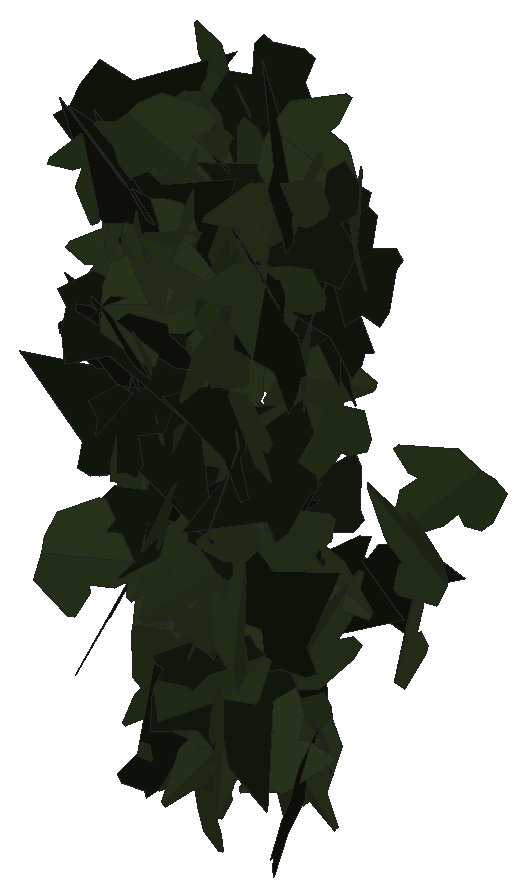
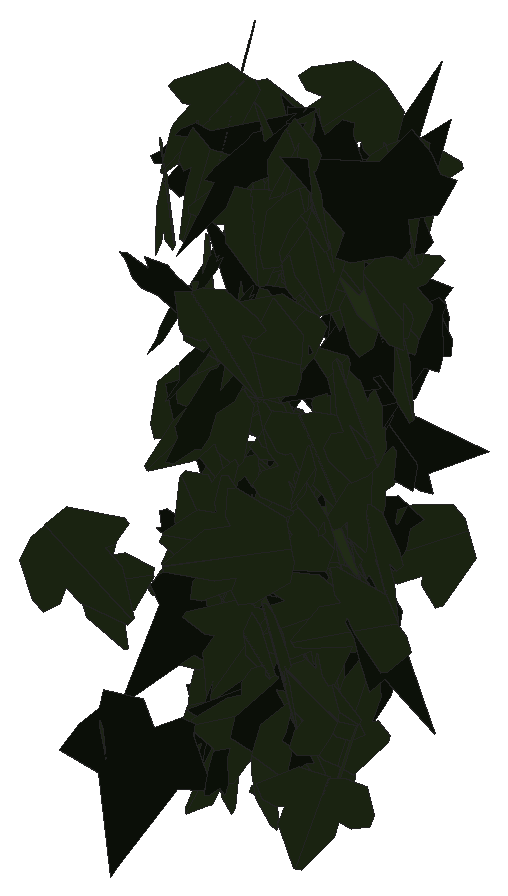
# SketchUp Ruby script. Lengths in inches.
U = 1.inch
M = Sketchup.active_model
def pt(a) = Geom::Point3d.new(a.map { |v| v * U })
def face(e, loops, mat)
  f = e.add_face(loops[0].map { |a| pt(a) })
  loops[1..].each { |l| e.add_face(l.map { |a| pt(a) }).erase! }
  f.material = f.back_material = mat if mat
  f
end
# faces: each face lists its corners as indices into pts; further lists are holes
def faces(e, pts, list, mat = nil) = list.each { |f| face(e, (f[0].is_a?(Array) ? f : [f]).map { |l| l.map { |i| pts[i] } }, mat) }
# xy, xz, yz: faces in a plane at the given z, y or x. An outline is a flat list of corners, or four numbers for a rectangle; further outlines are holes
def ring(l) = l.size == 4 ? [[l[0], l[1]], [l[2], l[1]], [l[2], l[3]], [l[0], l[3]]] : l.each_slice(2).to_a
def flat(e, list, mat, &to3) = list.each { |f| face(e, (f[0].is_a?(Array) ? f : [f]).map { |l| ring(l).map { |u, v| to3.(u, v) } }, mat) }
def xy(e, z, list, mat = nil) = flat(e, list, mat) { |x, y| [x, y, z] }
def xz(e, y, list, mat = nil) = flat(e, list, mat) { |x, z| [x, y, z] }
def yz(e, x, list, mat = nil) = flat(e, list, mat) { |y, z| [x, y, z] }
def lines(e, pts, list) = list.each { |a, b| e.add_line(pt(pts[a]), pt(pts[b])) }
# prism: a flat outline (further loops are holes) pulled along v
def prism(e, loops, v, mat = nil)
  f = face(e, loops, mat); d = Geom::Vector3d.new(v.map { |x| x * U })
  f.pushpull(f.normal.samedirection?(d) ? d.length : -d.length)
end
def box(e, o, s, mat = nil) = prism(e, [[o, [o[0] + s[0], o[1], o[2]], [o[0] + s[0], o[1] + s[1], o[2]], [o[0], o[1] + s[1], o[2]]]], [0, 0, s[2]], mat)
def at(x, y, z, deg = 0) = Geom::Transformation.translation(pt([x, y, z])) * Geom::Transformation.rotation(ORIGIN, Z_AXIS, deg.degrees)
def axes(o, x, y, z) = Geom::Transformation.new([*x, 0, *y, 0, *z, 0, *pt(o).to_a, 1])
def part(name) = M.definitions.add(name)
# library, detail: a bought-in or finely detailed component or shape, given as its bounding box
def library(name, o, s) = part(name).tap { |d| box(d.entities, o, s) }
def detail(e, o, s) = box(e.add_group.entities, o, s)
def put(e, d, t, mat = nil) = e.add_instance(d, t).tap { |i| i.material = mat if mat }
def group(e, t, mat = nil) = e.add_group.tap { |g| g.transformation = t; g.material = mat if mat }.entities
root = M.entities
M.materials.add("efeu1").color = [18, 25, 13]
M.materials.add("efeu2").color = [43, 57, 29]
c1 = part("ivyleaf_9")
p = [[1.54,2.16,1.25],[1.36,2.04,1.19],[-0.21,0.99,0.68],[-0.71,1.11,0.82],[-0.85,0.86,0.67],[-0.8,0.17,0.21],
  [-0.9,-0.01,0.1],[-0.67,-0.16,-0.02],[-0.08,-0.08,-0.05],[-0.03,-0.6,-0.4],[0.65,-0.88,-0.66],[0.83,-0.6,-0.49],
  [1.29,-0.42,-0.43],[1.8125,-0.07,-0.26],[1.21,0.44,0.15]]
faces(c1.entities,p,[[0,1,2,3,4,5,6,7,8,9,10,11,12,13,14]],"efeu1")
c2 = part("ivyleaf_10")
p = [[0,0.5,-0.03],[-0.0625,2.02,-0.43],[-0.19,2.01,-0.46],[-0.54,1.05,-0.29],[-0.52,0.625,-0.18],[-0.83,0.76,-0.28],
  [-1.16,0.64,-0.33],[-1.15,0.33,-0.24],[-0.77,-0.39,0.02],[-0.3,-0.51,0.16],[0.04,-0.48,0.23],[-0.02,2.01,-0.4375],
  [-0.06,2.01,-0.43],[0.04,-0.49,0.23],[0.67,-0.49,0.14],[1.38,0.36,-0.2],[1.375,0.51,-0.24],[0.81,0.65,-0.19],
  [0.62,0.59,-0.15],[0.6,1.09,-0.28],[0.5,1.23,-0.31]]
faces(c2.entities,p,[[0,1,2,3,4,5,6,7,8,9,10],[11,12,0,13,14,15,16,17,18,19,20]],"efeu2")
put(root,c1,axes([26.66,224.62,208.91],[-0.32247,0.29396,-0.24413],[0.18066,-0.16419,-0.43635],[-0.33671,-0.36963,-0.00032]))
put(root,c2,axes([26.38,225.71,207.47],[0.36727,0.30466,0.14933],[0.11088,0.10021,-0.47714],[-0.32066,0.38359,0.00605]))
put(root,c1,axes([26.95,224.11,210.61],[-0.14975,0.07294,0.47144],[-0.41443,0.22483,-0.16642],[-0.23627,-0.4406,-0.00688]))
put(root,c2,axes([26.24,225.02,209.12],[0.16854,0.09885,0.46024],[0.40926,0.21078,-0.19514],[-0.2326,0.44249,-0.00986]))
put(root,c2,axes([26.69,224.51,209.83],[0.35731,-0.28348,-0.20487],[-0.12645,0.16836,-0.4535],[0.3261,0.37589,0.04862]))
put(root,c1,axes([26.35,224.49,213.49],[0.01271,-0.0227,0.49932],[0.47252,0.1634,-0.0046],[-0.16297,0.472,0.0256]))
put(root,c2,axes([26.74,224.15,213.72],[-0.17009,-0.46109,0.09202],[-0.03319,-0.08584,-0.49146],[0.46901,-0.17329,-0.0014]))
put(root,c2,axes([26.79,224.35,212.43],[-0.15202,-0.37316,0.29604],[-0.05824,-0.29386,-0.40032],[0.47276,-0.15619,0.04588]))
put(root,c2,axes([26.99,223.97,211.8],[-0.29436,0.07852,0.39646],[-0.3811,0.10939,-0.30462],[-0.13458,-0.48153,-0.00455]))
put(root,c2,axes([26.71,225.32,208.11],[0.1669,-0.368,0.29448],[-0.11796,0.26984,0.40407],[-0.45632,-0.20435,0.00325]))
put(root,c2,axes([26.63,224.75,210.91],[0.12839,-0.48002,0.05564],[-0.00091,0.05733,0.4967],[-0.48323,-0.12764,0.01385]))
put(root,c1,axes([26.7,223.81,212],[0.43165,-0.00238,-0.25233],[-0.25233,-0.00072,-0.43166],[0.00169,0.49999,-0.00182]))
put(root,c2,axes([26.54,223.61,209.36],[-0.07018,-0.11217,-0.48218],[0.39074,0.28648,-0.12351],[0.30397,-0.39415,0.04745]))
put(root,c2,axes([26.8125,224.88,207.56],[-0.08774,-0.37373,-0.32035],[-0.08605,-0.30875,0.38376],[-0.48466,0.12247,-0.01014]))
put(root,c2,axes([26.75,224.52,210.34],[0.03372,0.48819,-0.10261],[-0.01362,-0.10191,-0.48932],[-0.49868,0.0358,0.00643]))
put(root,c2,axes([26.53,226.45,210.49],[0.09097,0.00084,0.49165],[0.31999,0.3795,-0.05985],[-0.37327,0.32554,0.06851]))
put(root,c2,axes([26.92,225.83,209.22],[0.29573,-0.36078,-0.17996],[-0.11311,0.13997,-0.46649],[0.38698,0.31662,0.00117]))
put(root,c2,axes([26.6875,225.03,207.22],[-0.18584,0.19109,0.42302],[0.27247,-0.324,0.26606],[0.3758,0.32941,0.01629]))
put(root,c2,axes([26.91,225.19,213.4],[-0.15695,-0.37328,0.2933],[0.02865,-0.3158,-0.38659],[0.47386,-0.10454,0.12052]))
put(root,c1,axes([27.03,223.9375,212.95],[0.2348,-0.23037,0.37656],[-0.26863,0.26389,0.32894],[-0.35029,-0.35678,0.00016]))
put(root,c2,axes([26.97,225.26,213.63],[-0.23941,-0.43009,0.08777],[-0.0319,-0.08266,-0.49209],[0.4378,-0.24122,0.01214]))
put(root,c1,axes([26.96,224.13,213.37],[0.30114,-0.39567,0.05256],[-0.03143,0.04213,0.49723],[-0.39791,-0.30277,0.0005]))
put(root,c1,axes([27.02,223.77,211.93],[0.3575,0.26132,-0.23218],[-0.19488,-0.1267,-0.44268],[-0.29019,0.40702,0.01126]))
put(root,c2,axes([27.11,224.91,212.73],[-0.13222,-0.24673,-0.4143],[-0.20204,-0.36171,0.2799],[-0.43783,0.24143,-0.00405]))
put(root,c2,axes([27.3,225.08,214.12],[-0.31633,0.10684,0.37219],[-0.37553,0.03252,-0.32851],[-0.0944,-0.48737,0.05967]))
put(root,c2,axes([26.75,224.58,212.34],[0.08372,-0.3231,-0.37229],[0.26335,-0.2899,0.31081],[-0.4167,-0.24812,0.12163]))
put(root,c1,axes([26.83,223.88,211.78],[0.30772,0.27236,0.28483],[0.21768,0.18378,-0.41091],[-0.32852,0.37689,-0.00547]))
put(root,c2,axes([27.07,224.59,209.125],[0.46562,-0.12968,-0.12799],[-0.12406,0.03161,-0.48333],[0.13345,0.48185,-0.00274]))
put(root,c2,axes([27.0625,225.07,211.06],[0.48055,0.09254,-0.10249],[-0.10018,-0.02176,-0.48938],[-0.09504,0.49088,-0.00237]))
put(root,c2,axes([26.74,224.11,213.19],[0.13021,-0.04117,0.48099],[0.4486,-0.17371,-0.13631],[0.17833,0.46704,-0.0083]))
put(root,c2,axes([27.15,224.48,210.84],[-0.0681,0.20334,0.45168],[-0.15786,0.42325,-0.21434],[-0.46951,-0.1718,0.00655]))
put(root,c2,axes([27.15,224.3125,209.64],[0.44624,-0.19654,-0.11065],[-0.10116,0.04485,-0.4876],[0.20159,0.45756,0.00027]))
put(root,c2,axes([27.14,225.11,207.89],[0.48342,0.05597,-0.11477],[-0.11472,-0.00696,-0.48661],[-0.05606,0.49681,0.00611]))
put(root,c2,axes([27.45,225.1,208.28],[0.1991,-0.04854,-0.45607],[-0.45201,0.0635,-0.20409],[0.07773,0.49357,-0.01859]))
put(root,c2,axes([27.05,225.79,207.6],[0.13461,-0.29777,0.37844],[0.18074,-0.33297,-0.32628],[0.44633,0.22464,0.018]))
put(root,c1,axes([26.97,223.95,212.22],[-0.11579,-0.28341,-0.39531],[0.13775,0.37062,-0.30605],[0.4665,-0.17978,-0.00775]))
put(root,c2,axes([27.35,224.64,211.24],[0.36899,-0.05366,0.33312],[-0.3307,0.04043,0.37283],[-0.06695,-0.49546,-0.00566]))
put(root,c2,axes([26.89,224.72,209.55],[0.16943,-0.27801,-0.37947],[0.26978,-0.273,0.32046],[-0.38537,-0.31334,0.05749]))
put(root,c2,axes([26.875,225.11,209.07],[-0.27082,-0.01515,-0.42003],[0.41997,0.0103,-0.27114],[0.01687,-0.49966,0.00715]))
put(root,c2,axes([27.26,224.39,209.98],[0.15567,-0.46179,-0.11189],[-0.03442,0.10648,-0.48732],[0.4739,0.15942,0.00137]))
put(root,c2,axes([27.11,225,208.39],[0.35133,-0.30438,0.18417],[0.13781,-0.1222,-0.46484],[0.32798,0.37739,-0.00198]))
put(root,c2,axes([27.01,225.07,213.54],[0.30215,-0.18447,0.3531],[0.32464,-0.14285,-0.35243],[0.2309,0.44223,0.03344]))
put(root,c2,axes([27.59,224.39,209.08],[-0.31412,-0.10851,0.37357],[-0.35757,-0.10858,-0.3322],[0.15322,-0.47585,-0.00939]))
put(root,c1,axes([27.04,224.21,210.85],[-0.16668,-0.16086,-0.44311],[0.33106,0.29463,-0.23149],[0.33558,-0.37056,0.00829]))
put(root,c1,axes([27.06,224.25,209.89],[-0.02119,-0.14971,-0.47659],[0.16131,0.44941,-0.14835],[0.47279,-0.16004,0.02925]))
put(root,c1,axes([27.2,224.97,207.67],[0.09233,0.06535,0.48704],[0.35486,0.33394,-0.11208],[-0.33993,0.36635,0.01528]))
put(root,c2,axes([27.02,225.05,209.92],[0.13656,-0.06296,-0.47685],[0.41465,-0.2358,0.14988],[-0.24376,-0.43639,-0.01219]))
put(root,c2,axes([27.21,225.24,212.29],[0.18438,0.33099,0.32627],[0.14306,0.29354,-0.37864],[-0.4422,0.23298,0.01355]))
put(root,c2,axes([27.31,224.48,207.34],[-0.0789,0.12259,0.47828],[0.19257,-0.43834,0.14412],[0.45463,0.20695,0.02195]))
put(root,c2,axes([27.39,224.79,214],[-0.1864,0.46079,0.05413],[-0.02106,0.04987,-0.49706],[-0.46348,-0.18758,0.00081]))
put(root,c2,axes([27.37,224.69,210.33],[-0.02032,-0.45723,0.20133],[0.02404,0.20036,0.45747],[-0.49901,0.02827,0.01384]))
put(root,c2,axes([27.34,224.63,210.57],[-0.31041,-0.24057,-0.30946],[0.23259,0.2047,-0.39243],[0.31551,-0.38759,-0.01517]))
put(root,c2,axes([27.12,223.84,212.21],[0.00608,-0.04671,-0.49778],[0.45921,0.19739,-0.01292],[0.19772,-0.45701,0.0453]))
put(root,c1,axes([27.54,224.26,213.83],[0.36088,0.11412,-0.32672],[-0.32167,-0.06352,-0.37749],[-0.12766,0.48264,0.02757]))
put(root,c2,axes([27.4375,225.47,207.89],[0.02541,0.12411,-0.48368],[0.12532,0.46722,0.12647],[0.48337,-0.12766,-0.00736]))
put(root,c2,axes([27.62,225.99,212.64],[0.44038,-0.07107,-0.22587],[-0.22418,0.02837,-0.44602],[0.07622,0.49411,-0.00688]))
put(root,c1,axes([27.47,224.09,207.21],[0.16483,0.28702,0.37477],[-0.25902,-0.27687,0.32596],[0.39464,-0.3016,0.05741]))
put(root,c2,axes([27.45,225.83,209.93],[0.0848,-0.25818,0.41971],[-0.02272,0.42338,0.26502],[-0.49223,-0.06402,0.06008]))
put(root,c2,axes([27.16,225.45,212.03],[-0.02105,-0.0175,0.49925],[0.44755,0.22134,0.02663],[-0.22194,0.448,0.00635]))
put(root,c2,axes([27.32,224.74,209.61],[0.25451,0.25694,0.34526],[0.22832,0.25941,-0.36135],[-0.36482,0.3416,0.01471]))
put(root,c2,axes([27.42,224.3,212.57],[-0.39143,0.19549,-0.242],[0.2207,-0.09962,-0.43745],[-0.21925,-0.44929,-0.0083]))
put(root,c2,axes([27.36,223.85,214.19],[-0.33602,-0.07922,-0.36168],[0.35792,0.05553,-0.34469],[0.09478,-0.49055,0.01939]))
put(root,c1,axes([27.34,224.02,212.88],[-0.12516,0.02953,0.48318],[0.38729,-0.29329,0.11825],[0.29041,0.40386,0.05054]))
put(root,c2,axes([27.26,223.91,212.87],[-0.05179,-0.02453,-0.49671],[0.46638,-0.17576,-0.03995],[-0.17264,-0.46745,0.04108]))
put(root,c1,axes([27.64,226.875,208.21],[0.33413,0.35247,-0.11886],[-0.08165,-0.08637,-0.48567],[-0.36289,0.34396,-0.00015]))
put(root,c1,axes([27.39,224.52,209.55],[0.27225,0.13782,0.39609],[0.32915,0.22241,-0.30363],[-0.25988,0.42607,0.03038]))
put(root,c2,axes([27.45,224.82,210.6875],[0.43227,-0.12582,-0.21752],[0.20811,-0.06333,0.4502],[-0.14084,-0.47975,-0.00238]))
put(root,c1,axes([27.56,225.23,214.18],[0.19724,-0.29109,-0.35547],[-0.11217,0.34463,-0.34445],[0.44555,0.21563,0.07065]))
put(root,c2,axes([27.91,224.3,212.73],[-0.20826,-0.15079,-0.42882],[-0.26357,-0.34424,0.24906],[-0.37035,0.32979,0.06389]))
put(root,c2,axes([27.66,225.21,213.47],[0.45445,0.20775,0.01787],[0.01301,0.01452,-0.49962],[-0.20811,0.45456,0.00779]))
put(root,c2,axes([27.56,225.29,208.75],[0.3027,0.31652,0.24123],[0.17024,0.17096,-0.43794],[-0.35971,0.34726,-0.00427]))
put(root,c2,axes([27.76,224.5,213.66],[0.06388,0.29533,-0.39837],[-0.07105,-0.39207,-0.30205],[-0.49079,0.0952,-0.00812]))
put(root,c2,axes([27.83,225.82,210.17],[0.04879,0.38916,-0.31012],[-0.00186,0.31175,0.39091],[0.49761,-0.03699,0.03187]))
put(root,c2,axes([28.01,225.3,209.04],[0.32319,-0.10633,-0.36639],[-0.32469,0.17546,-0.33732],[0.20031,0.45597,0.04436]))
put(root,c2,axes([27.89,224.37,210.47],[0.26488,-0.40629,-0.12152],[-0.06714,0.10129,-0.48501],[0.41872,0.27326,-0.0009]))
put(root,c2,axes([27.5625,224.33,206.77],[-0.2588,0.02355,0.42716],[0.40892,-0.13312,0.25508],[0.12574,0.48138,0.04964]))
put(root,c1,axes([27.86,224.65,210.65],[0.23539,-0.4283,-0.10561],[0.05866,-0.08825,0.48864],[-0.43721,-0.24243,0.0087]))
put(root,c1,axes([28.24,225.4,209.4375],[-0.45474,-0.08495,-0.18972],[-0.18679,-0.03325,0.46261],[-0.09121,0.49161,-0.0015]))
put(root,c2,axes([27.92,224.31,208.99],[0.04676,-0.46604,0.17499],[0.03804,-0.1719,-0.46798],[0.49635,0.05707,0.01938]))
put(root,c1,axes([27.59,225.94,211.48],[0.18573,-0.37886,0.26826],[0.17236,-0.21201,-0.41874],[0.43104,0.24802,0.05185]))
put(root,c2,axes([28.03,224.36,207.65],[-0.08885,-0.28885,0.39833],[-0.06229,-0.39492,-0.30027],[0.48808,-0.10298,0.03419]))
put(root,c1,axes([27.7,224.88,211.84],[-0.17637,0.16439,0.43803],[0.32334,-0.29551,0.24109],[0.33815,0.36831,-0.00207]))
put(root,c2,axes([28,224.03,212.4375],[0.08458,-0.15469,0.46789],[-0.16382,0.4389,0.17472],[-0.46477,-0.18286,0.02357]))
put(root,c1,axes([27.73,225.76,212.13],[0.17746,-0.45434,0.10992],[0.05498,-0.09647,-0.48751],[0.4642,0.18511,0.01572]))
put(root,c1,axes([28.14,224.89,209.64],[-0.2407,0.36006,-0.24984],[0.13416,-0.21082,-0.43308],[-0.41721,-0.27552,0.00488]))
put(root,c2,axes([28.09,224.42,207.81],[0.12149,-0.48435,-0.02538],[-0.00526,0.02484,-0.49935],[0.48499,0.1216,0.00094]))
put(root,c2,axes([28.09,223.98,212.13],[0.00204,-0.42267,-0.2671],[0.05102,0.26589,-0.42036],[0.49739,-0.02554,0.04422]))
put(root,c2,axes([27.82,224.68,213.62],[-0.09251,0.06195,-0.48745],[0.29904,-0.38648,-0.10587],[-0.38989,-0.31112,0.03445]))
put(root,c2,axes([28.15,225.03,207.1],[0.01967,-0.14105,-0.47929],[-0.0166,0.47921,-0.14171],[0.49934,0.02149,0.01417]))
put(root,c2,axes([28.12,226.8125,207.38],[0.35656,-0.32509,0.13107],[-0.0962,0.08903,0.48251],[-0.33706,-0.36931,0.00095]))
put(root,c2,axes([28.05,224.875,209.44],[-0.22937,0.42218,-0.13838],[0.06926,-0.11985,-0.48046],[-0.43885,-0.23958,-0.0035]))
put(root,c2,axes([28.17,224.3,212.52],[-0.04038,-0.34842,-0.35633],[0.03216,0.35493,-0.3507],[0.49733,-0.05124,-0.00625]))
put(root,c1,axes([27.77,225.4375,207.56],[0.20988,-0.02548,-0.4531],[0.44833,-0.06577,0.21137],[-0.07037,-0.495,-0.00476]))
put(root,c2,axes([28.05,225.24,211.13],[-0.11051,-0.22254,-0.43389],[0.21006,0.37977,-0.24828],[0.44007,-0.23717,0.00956]))
put(root,c2,axes([28.5,224.91,207.36],[0.05805,-0.01432,-0.49641],[-0.38503,0.31436,-0.0541],[0.31365,0.38855,0.02547]))
put(root,c2,axes([28.04,223.81,207.91],[-0.28973,-0.30679,0.26821],[0.1934,0.18615,0.42184],[-0.35868,0.34818,0.0108]))
put(root,c2,axes([28.03,224.44,210.98],[-0.30722,0.27725,-0.28063],[0.21354,-0.1822,-0.41377],[-0.33169,-0.37408,-0.00646]))
put(root,c1,axes([28.17,225.36,207.34],[-0.01871,-0.08629,0.49214],[-0.11287,-0.47903,-0.08828],[0.48674,-0.1144,-0.00155]))
put(root,c1,axes([28.11,223.96,208.49],[-0.17635,-0.29136,-0.36607],[0.18878,0.31364,-0.34058],[0.42809,-0.25833,-0.00062]))
put(root,c1,axes([28.29,225.2,208.86],[0.00111,-0.01941,-0.49962],[-0.2074,0.45459,-0.01812],[0.45495,0.20729,-0.00704]))
put(root,c2,axes([28.4,224.26,209.81],[-0.47473,-0.15525,0.02309],[-0.01982,-0.01369,-0.49942],[0.1557,-0.47509,0.00684]))
put(root,c2,axes([28.23,223.99,208.0625],[-0.05027,0.40076,-0.29473],[0.04509,-0.29134,-0.40384],[-0.49542,-0.06718,-0.00685]))
put(root,c2,axes([27.98,225.1875,209.21],[0.21231,0.03492,0.45134],[0.41735,0.17798,-0.21009],[-0.17533,0.46595,0.04642]))
put(root,c2,axes([28.51,224.96,207.46],[0.04665,0.12104,-0.48288],[-0.1665,-0.45327,-0.1297],[-0.46915,0.1729,-0.00198]))
put(root,c1,axes([28.42,223.92,213.26],[0.40117,-0.04263,-0.29537],[-0.29136,0.0511,-0.40311],[0.06456,0.49555,0.01616]))
put(root,c1,axes([28.74,224.3125,210.79],[-0.48061,0.11443,0.07697],[-0.07504,0.01713,-0.49404],[-0.1157,-0.48643,0.00071]))
put(root,c2,axes([28.61,224.89,210.95],[-0.32229,-0.35931,0.13047],[-0.08617,-0.09797,-0.48268],[0.37243,-0.33361,0.00123]))
put(root,c2,axes([28.61,223.52,209.05],[-0.02815,0.24753,-0.43352],[-0.11527,0.41925,0.24686],[0.48572,0.11384,0.03346]))
put(root,c1,axes([28.64,225.58,212.52],[-0.4928,-0.02762,-0.07988],[0.07975,0.00457,-0.49358],[0.02799,-0.49922,-0.0001]))
put(root,c2,axes([28.46,224.875,208.25],[0.01488,-0.42291,0.26632],[-0.01428,0.26597,0.42315],[-0.49957,-0.0202,-0.00416]))
put(root,c2,axes([28.3,224.74,207.46],[-0.30091,0.18012,-0.35639],[0.31118,-0.17388,-0.35062],[-0.25024,-0.43281,-0.00745]))
put(root,c2,axes([28.375,225,211.67],[0.13951,-0.29596,-0.37808],[0.15561,-0.3446,0.32716],[-0.45423,-0.20895,-0.00404]))
put(root,c1,axes([28.47,225.35,212.05],[0.28043,-0.35152,-0.21861],[0.13514,-0.17185,0.44967],[-0.39128,-0.31129,-0.00137]))
put(root,c2,axes([28.68,224.16,213.72],[-0.26756,-0.41732,0.0652],[-0.03382,-0.05576,-0.49573],[0.42103,-0.26969,0.00161]))
put(root,c2,axes([28.7,223.99,212.89],[-0.37318,-0.32767,0.05808],[-0.04044,-0.04197,-0.49659],[0.33031,-0.37533,0.00482]))
put(root,c2,axes([28.48,224.13,207.57],[0.47649,0.1149,-0.09875],[0.09571,0.02431,0.49015],[0.11744,-0.48601,0.00118]))
put(root,c2,axes([28.65,224.6,213.57],[-0.05111,-0.38646,-0.31311],[0.03683,0.31096,-0.38981],[0.49602,-0.06291,-0.00332]))
put(root,c1,axes([28.91,224.74,213.31],[-0.20209,-0.39757,-0.22604],[-0.07966,-0.21275,0.44541],[-0.45035,0.21604,0.02265]))
put(root,c1,axes([28.74,224.27,213.62],[0.07596,-0.36011,0.33846],[0.02291,0.34463,0.36153],[-0.49366,-0.03941,0.06886]))
put(root,c2,axes([28.54,224.53,214.14],[0.05501,0.35849,0.34418],[0.06699,0.33777,-0.36252],[-0.49243,0.08599,-0.01087]))
put(root,c2,axes([29.05,225.97,209.04],[-0.19791,0.12137,-0.44283],[-0.39405,0.20265,0.23165],[0.23571,0.44068,0.01544]))
put(root,c1,axes([28.95,224.04,207.3],[-0.08899,0.05298,-0.48916],[-0.40689,0.27155,0.10343],[0.27662,0.41648,-0.00522]))
put(root,c2,axes([29.03,226.56,209.71],[-0.26019,-0.23506,0.35644],[-0.27083,-0.23182,-0.35058],[0.33008,-0.37551,-0.00669]))
put(root,c1,axes([29.07,223.74,212.7],[0.05232,0.02508,-0.49662],[-0.49328,-0.06042,-0.05502],[-0.06277,0.4957,0.01842]))
put(root,c2,axes([29.08,224.89,213.06],[-0.02374,0.01868,0.49909],[-0.41958,0.27027,-0.03008],[-0.2709,-0.42024,0.00284]))
put(root,c1,axes([28.51,224.17,208.99],[-0.09452,0.07951,0.4845],[0.349,-0.33617,0.12326],[0.34535,0.36148,0.00805]))
